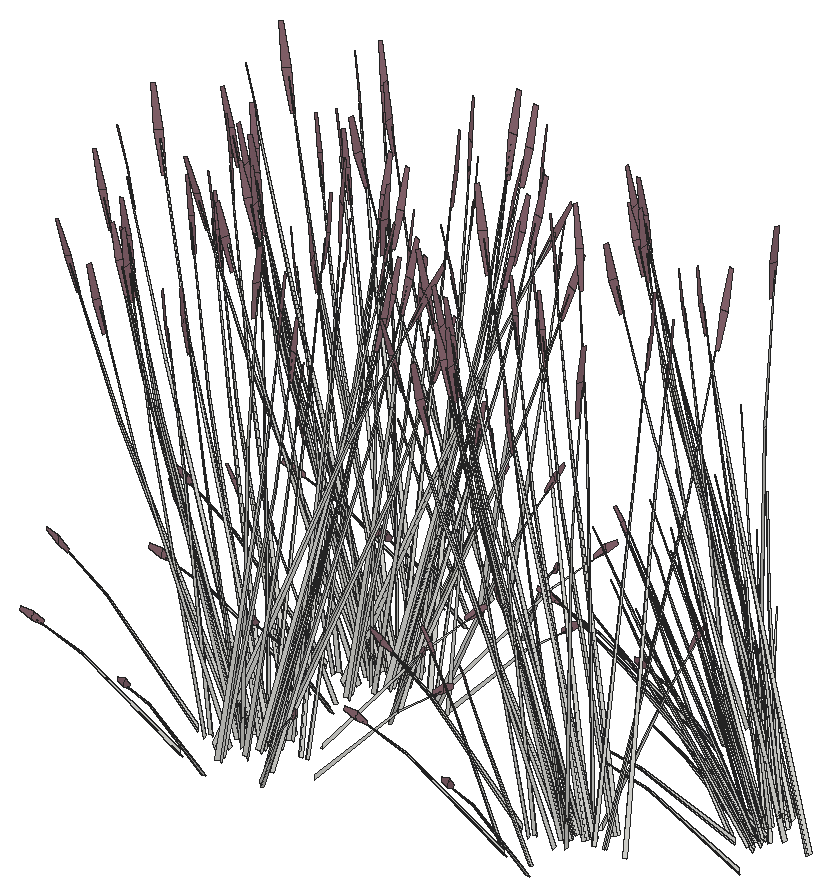
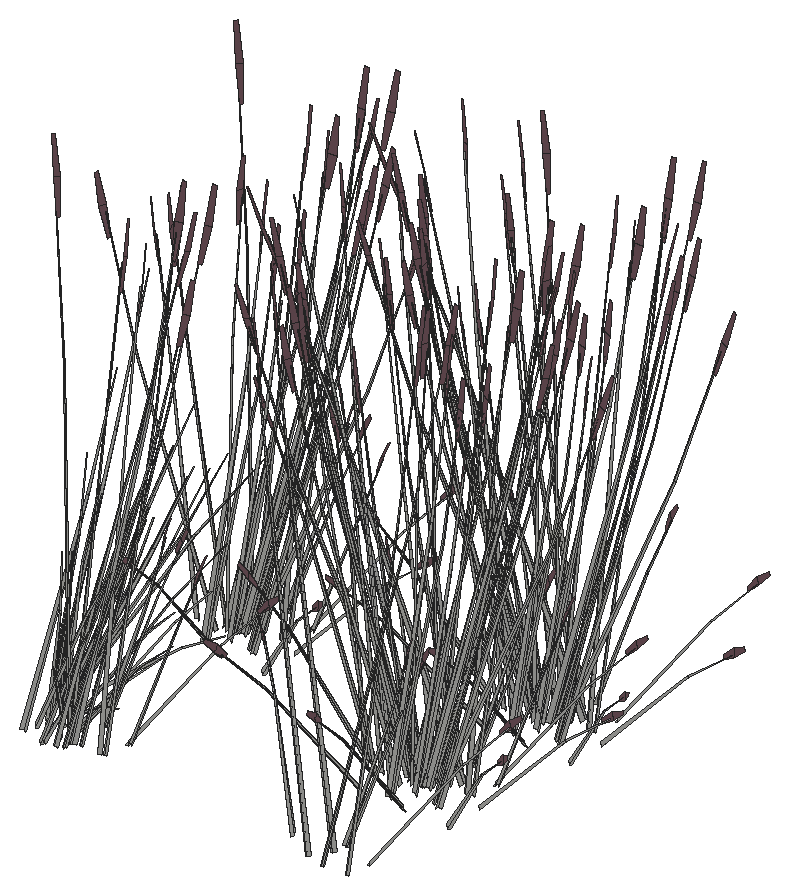
# SketchUp Ruby script. Lengths in inches.
U = 1.inch
M = Sketchup.active_model
def pt(a) = Geom::Point3d.new(a.map { |v| v * U })
def face(e, loops, mat)
  f = e.add_face(loops[0].map { |a| pt(a) })
  loops[1..].each { |l| e.add_face(l.map { |a| pt(a) }).erase! }
  f.material = f.back_material = mat if mat
  f
end
# faces: each face lists its corners as indices into pts; further lists are holes
def faces(e, pts, list, mat = nil) = list.each { |f| face(e, (f[0].is_a?(Array) ? f : [f]).map { |l| l.map { |i| pts[i] } }, mat) }
# xy, xz, yz: faces in a plane at the given z, y or x. An outline is a flat list of corners, or four numbers for a rectangle; further outlines are holes
def ring(l) = l.size == 4 ? [[l[0], l[1]], [l[2], l[1]], [l[2], l[3]], [l[0], l[3]]] : l.each_slice(2).to_a
def flat(e, list, mat, &to3) = list.each { |f| face(e, (f[0].is_a?(Array) ? f : [f]).map { |l| ring(l).map { |u, v| to3.(u, v) } }, mat) }
def xy(e, z, list, mat = nil) = flat(e, list, mat) { |x, y| [x, y, z] }
def xz(e, y, list, mat = nil) = flat(e, list, mat) { |x, z| [x, y, z] }
def yz(e, x, list, mat = nil) = flat(e, list, mat) { |y, z| [x, y, z] }
def lines(e, pts, list) = list.each { |a, b| e.add_line(pt(pts[a]), pt(pts[b])) }
# prism: a flat outline (further loops are holes) pulled along v
def prism(e, loops, v, mat = nil)
  f = face(e, loops, mat); d = Geom::Vector3d.new(v.map { |x| x * U })
  f.pushpull(f.normal.samedirection?(d) ? d.length : -d.length)
end
def box(e, o, s, mat = nil) = prism(e, [[o, [o[0] + s[0], o[1], o[2]], [o[0] + s[0], o[1] + s[1], o[2]], [o[0], o[1] + s[1], o[2]]]], [0, 0, s[2]], mat)
def at(x, y, z, deg = 0) = Geom::Transformation.translation(pt([x, y, z])) * Geom::Transformation.rotation(ORIGIN, Z_AXIS, deg.degrees)
def axes(o, x, y, z) = Geom::Transformation.new([*x, 0, *y, 0, *z, 0, *pt(o).to_a, 1])
def part(name) = M.definitions.add(name)
# library, detail: a bought-in or finely detailed component or shape, given as its bounding box
def library(name, o, s) = part(name).tap { |d| box(d.entities, o, s) }
def detail(e, o, s) = box(e.add_group.entities, o, s)
def put(e, d, t, mat = nil) = e.add_instance(d, t).tap { |i| i.material = mat if mat }
def group(e, t, mat = nil) = e.add_group.tap { |g| g.transformation = t; g.material = mat if mat }.entities
root = M.entities
M.materials.add("LightPink_Translucent").color = [144, 107, 117]
c1 = part("blade")
p = [[2.15,0.21,22],[0,0.17,0],[0.09,0.45,0],[2.18,0.31,22],[2.29,0.31,22],[0.38,0.45,0],
  [2.48,0.24,33],[2.49,0.24,33],[2.48,0.22,33]]
faces(c1.entities,p,[[0,1,2,3],[4,5,2,3],[6,3,4,7],[8,0,3,6]])
c2 = part("seeds")
p = [[0.3,-0.1,1.38],[-0.01,-0.03,1.59],[-0.01,-0.03,0.03],[0.14,-0.07,-0.07],[0.29,-0.03,3],[0.15,0.01,3.11]]
faces(c2.entities,p,[[0,1,2,3],[1,0,4,5]],"LightPink_Translucent")
c3 = part("blade with seeds")
put(c3.entities,c1,at(0,0,0))
put(c3.entities,c2,axes([2.4,0.25,30.99],[1.5799,-0.05474,1.17369],[-0.12525,1.92788,0.29478],[-0.07173,-0.02425,1.56792]))
c4 = part("blade with seeds\#1")
put(c4.entities,c1,at(0,0,0))
put(root,c3,axes([24.625,21.875,43.74],[0.03108,0.16322,1.76342],[-0.62654,0.85237,-0.26939],[-0.44504,-0.04296,0.30037]))
put(root,c3,axes([24.29,26.44,43.74],[0.16438,0.10347,1.76342],[0.27873,0.95868,-0.26939],[-0.36432,0.20444,0.30037]))
put(root,c3,axes([26.17,37.93,43.49],[0.03108,0.16322,1.76342],[-0.62654,0.85237,-0.26939],[-0.44504,-0.04296,0.30037]))
put(root,c3,axes([25.83,42.51,43.49],[0.16438,0.10347,1.76342],[0.27873,0.95868,-0.26939],[-0.36432,0.20444,0.30037]))
put(root,c3,axes([28.72,23.35,44.31],[-1.27479,-0.1698,-0.62353],[0.26901,-1.04736,-0.16365],[-0.38043,-0.12691,1.37633]))
put(root,c3,axes([27.05,25.34,44.27],[-1.14694,-0.51783,-0.49651],[0.68554,-0.92854,0],[-0.26122,-0.11794,1.57504]))
put(root,c3,axes([26.55,17.62,43.74],[-0.11871,0.13643,1.76342],[-1.19964,0.29415,-0.26939],[-0.2898,-0.26759,0.30037]))
put(root,c3,axes([30.27,39.41,44.06],[-1.27479,-0.1698,-0.62353],[0.26901,-1.04736,-0.16365],[-0.38043,-0.12691,1.37633]))
put(root,c3,axes([27.79,52.71,43.49],[-0.11871,0.13643,1.76342],[-1.19964,0.29415,-0.26939],[-0.2898,-0.26759,0.30037]))
put(root,c3,axes([28.59,41.4,44.02],[-1.14694,-0.51783,-0.49651],[0.68554,-0.92854,0],[-0.26122,-0.11794,1.57504]))
put(root,c3,axes([28.09,33.68,43.49],[-0.11871,0.13643,1.76342],[-1.19964,0.29415,-0.26939],[-0.2898,-0.26759,0.30037]))
put(root,c3,axes([30.17,23.51,44.92],[-1.23732,0.68758,-0.29095],[-0.8228,-0.97154,-0.50002],[-0.30528,-0.09867,1.59708]))
put(root,c3,axes([27.37,24.95,44.28],[-0.28787,-0.90242,-0.30978],[1.14332,-0.25625,0.30978],[-0.23049,-0.10406,1.38974]))
put(root,c3,axes([30.99,24.26,44.31],[-0.82544,0.77843,-0.62353],[-1.0254,-0.70586,-0.16365],[-0.33076,0.19418,1.37633]))
put(root,c3,axes([27.34,34.21,44.13],[-0.35352,0.84566,-0.03893],[-1.08806,-0.26014,-0.17649],[-0.1652,-0.13832,0.58215]))
put(root,c3,axes([31.56,23.82,44.72],[-1.19666,-0.83357,-0.25192],[1.00694,-0.93603,0.5513],[-0.32224,0.09751,1.68216]))
put(root,c3,axes([31.71,39.57,44.67],[-1.23732,0.68758,-0.29095],[-0.8228,-0.97154,-0.50002],[-0.30528,-0.09867,1.59708]))
put(root,c3,axes([29.38,23.02,44.46],[-0.73619,-0.86927,-0.44739],[1.11511,-0.61213,0.21531],[-0.23824,-0.10756,1.43643]))
put(root,c3,axes([28.91,41.01,44.03],[-0.28787,-0.90242,-0.30978],[1.14332,-0.25625,0.30978],[-0.23049,-0.10406,1.38974]))
put(root,c3,axes([30.95,23.64,44.46],[-1.33077,0.06393,-0.44739],[-0.12035,-1.06125,0.21531],[-0.23824,0.10756,1.43643]))
put(root,c3,axes([32.53,40.32,44.06],[-0.82544,0.77843,-0.62353],[-1.0254,-0.70586,-0.16365],[-0.33076,0.19418,1.37633]))
put(root,c3,axes([33.1,39.88,44.46],[-1.19666,-0.83357,-0.25192],[1.00694,-0.93603,0.5513],[-0.32224,0.09751,1.68216]))
put(root,c3,axes([30.93,39.08,44.21],[-0.73619,-0.86927,-0.44739],[1.11511,-0.61213,0.21531],[-0.23824,-0.10756,1.43643]))
put(root,c3,axes([32.35,26.38,44.27],[-1.14694,0.51783,-0.49651],[-0.68554,-0.92854,0],[-0.26122,0.11794,1.57504]))
put(root,c3,axes([25.56,21.22,44.27],[0,-1.03566,-0.49651],[1.37109,0,0],[0,-0.23588,1.57504]))
put(root,c3,axes([32.5,39.7,44.21],[-1.33077,0.06393,-0.44739],[-0.12035,-1.06125,0.21531],[-0.23824,0.10756,1.43643]))
put(root,c3,axes([32.08,25.97,44.28],[-1.14332,-0.25625,-0.30978],[0.28787,-0.90242,0.30978],[-0.23049,0.10406,1.38974]))
put(root,c3,axes([29.14,22.42,44.92],[-1.38012,-0.49416,-0.29095],[0.66454,-1.04299,-0.50002],[-0.04337,-0.25608,1.59708]))
put(root,c3,axes([31.03,39.58,44.4375],[0.32481,-1.2272,-0.23429],[1.54007,0.21392,0.51271],[-0.26911,-0.16947,1.5644]))
put(root,c3,axes([31.88,23.36,44.92],[0.1428,1.18174,-0.29095],[-1.48733,0.07145,-0.50002],[-0.26191,0.15741,1.59708]))
put(root,c3,axes([26.8,56.3125,44.02],[0,-1.03566,-0.49651],[1.37109,0,0],[0,-0.23588,1.57504]))
put(root,c3,axes([28.53,21.37,44.35],[-0.50328,-1.06202,-0.69835],[1.44974,-0.38248,-0.18329],[-0.05563,-0.35963,1.54149]))
put(root,c3,axes([33.89,42.44,44.02],[-1.14694,0.51783,-0.49651],[-0.68554,-0.92854,0],[-0.26122,0.11794,1.57504]))
put(root,c3,axes([27.1,37.28,44.02],[0,-1.03566,-0.49651],[1.37109,0,0],[0,-0.23588,1.57504]))
put(root,c3,axes([26.15,21.25,44.28],[0.85545,-0.64616,-0.30978],[0.85545,0.64616,0.30978],[0,-0.20813,1.38974]))
put(root,c3,axes([33.625,42.03,44.03],[-1.14332,-0.25625,-0.30978],[0.28787,-0.90242,0.30978],[-0.23049,0.10406,1.38974]))
put(root,c3,axes([30.6875,38.48,44.67],[-1.38012,-0.49416,-0.29095],[0.66454,-1.04299,-0.50002],[-0.04337,-0.25608,1.59708]))
put(root,c3,axes([29.77,56.46,44.1],[-0.50328,-1.06202,-0.69835],[1.44974,-0.38248,-0.18329],[-0.05563,-0.35963,1.54149]))
put(root,c3,axes([33.43,39.42,44.67],[0.1428,1.18174,-0.29095],[-1.48733,0.07145,-0.50002],[-0.26191,0.15741,1.59708]))
put(root,c3,axes([30.07,37.43,44.1],[-0.50328,-1.06202,-0.69835],[1.44974,-0.38248,-0.18329],[-0.05563,-0.35963,1.54149]))
put(root,c3,axes([31.26,52.16,44.13],[-0.84686,0.59414,-0.03893],[-0.77596,-0.65071,-0.17649],[-0.05463,-0.18438,0.58215]))
put(root,c3,axes([27.69,37.31,44.03],[0.85545,-0.64616,-0.30978],[0.85545,0.64616,0.30978],[0,-0.20813,1.38974]))
put(root,c3,axes([31.55,33.13,44.13],[-0.84686,0.59414,-0.03893],[-0.77596,-0.65071,-0.17649],[-0.05463,-0.18438,0.58215]))
put(root,c3,axes([30.22,16.34,43.74],[-0.20555,0.03731,1.76342],[-1.13672,-0.42002,-0.26939],[0.01907,-0.35034,0.30037]))
put(root,c3,axes([29.29,21.65,44.46],[0.59459,-0.93321,-0.44739],[1.23546,0.44912,0.21531],[0,-0.21512,1.43643]))
put(root,c3,axes([29.36,26.54,43.74],[0.19833,-0.05635,1.76342],[1.19302,0.31018,-0.26939],[0.03489,0.3496,0.30037]))
put(root,c3,axes([31.47,51.43,43.49],[-0.20555,0.03731,1.76342],[-1.13672,-0.42002,-0.26939],[0.01907,-0.35034,0.30037]))
put(root,c3,axes([32.43,22.89,44.46],[-0.59459,0.93321,-0.44739],[-1.23546,-0.44912,0.21531],[0,0.21512,1.43643]))
put(root,c3,axes([31.77,32.4,43.49],[-0.20555,0.03731,1.76342],[-1.13672,-0.42002,-0.26939],[0.01907,-0.35034,0.30037]))
put(root,c3,axes([30.83,37.71,44.21],[0.59459,-0.93321,-0.44739],[1.23546,0.44912,0.21531],[0,-0.21512,1.43643]))
put(root,c3,axes([30.91,42.6,43.49],[0.19833,-0.05635,1.76342],[1.19302,0.31018,-0.26939],[0.03489,0.3496,0.30037]))
put(root,c3,axes([33.97,38.95,44.21],[-0.59459,0.93321,-0.44739],[-1.23546,-0.44912,0.21531],[0,0.21512,1.43643]))
put(root,c3,axes([35.57,23.29,44.28],[-0.85545,0.64616,-0.30978],[-0.85545,-0.64616,0.30978],[0,0.20813,1.38974]))
put(root,c3,axes([33.125,23.18,44.35],[0.44936,0.94823,-0.69212],[-1.29441,0.3415,-0.18165],[0.04967,0.32109,1.52773]))
put(root,c3,axes([29.83,21.18,44.92],[-0.1428,-1.18174,-0.29095],[1.48733,-0.07145,-0.50002],[0.26191,-0.15741,1.59708]))
put(root,c3,axes([32.57,22.12,44.92],[1.38012,0.49416,-0.29095],[-0.66454,1.04299,-0.50002],[0.04337,0.25608,1.59708]))
put(root,c3,axes([29.64,18.57,44.28],[1.14332,0.25625,-0.30978],[-0.28787,0.90242,0.30978],[0.23049,-0.10406,1.38974]))
put(root,c3,axes([37.12,39.35,44.03],[-0.85545,0.64616,-0.30978],[-0.85545,-0.64616,0.30978],[0,0.20813,1.38974]))
put(root,c3,axes([36.16,23.32,44.27],[0,1.03566,-0.49651],[-1.37109,0,0],[0,0.23588,1.57504]))
put(root,c3,axes([29.37,18.16,44.27],[1.14694,-0.51783,-0.49651],[0.68554,0.92854,0],[0.26122,-0.11794,1.57504]))
put(root,c3,axes([34.67,39.24,44.09],[0.44936,0.94823,-0.69212],[-1.29441,0.3415,-0.18165],[0.04967,0.32109,1.52773]))
put(root,c3,axes([31.38,37.24,44.67],[-0.1428,-1.18174,-0.29095],[1.48733,-0.07145,-0.50002],[0.26191,-0.15741,1.59708]))
put(root,c3,axes([34.12,38.18,44.67],[1.38012,0.49416,-0.29095],[-0.66454,1.04299,-0.50002],[0.04337,0.25608,1.59708]))
put(root,c3,axes([32.31,24.53,44.4375],[1.2866,-0.3514,-0.19198],[0.45209,1.01223,0.00008],[0.14202,-0.03884,1.73897]))
put(root,c3,axes([31.18,34.63,44.03],[1.14332,0.25625,-0.30978],[-0.28787,0.90242,0.30978],[0.23049,-0.10406,1.38974]))
put(root,c3,axes([30.61,53.25,44.02],[1.14694,-0.51783,-0.49651],[0.68554,0.92854,0],[0.26122,-0.11794,1.57504]))
put(root,c3,axes([37.7,39.38,44.02],[0,1.03566,-0.49651],[-1.37109,0,0],[0,0.23588,1.57504]))
put(root,c3,axes([30.91,34.22,44.02],[1.14694,-0.51783,-0.49651],[0.68554,0.92854,0],[0.26122,-0.11794,1.57504]))
put(root,c3,axes([32.33,21.52,44.46],[0.73619,0.86927,-0.44739],[-1.11511,0.61213,0.21531],[0.23824,0.10756,1.43643]))
put(root,c3,axes([30.73,20.28,44.31],[0.82544,-0.77843,-0.62353],[1.0254,0.70586,-0.16365],[0.33076,-0.19418,1.37633]))
put(root,c3,axes([33.85,40.59,44.18],[1.2866,-0.3514,-0.19198],[0.45209,1.01223,0.00008],[0.14202,-0.03884,1.73897]))
put(root,c3,axes([34.35,19.59,44.28],[0.28787,0.90242,-0.30978],[-1.14332,0.25625,0.30978],[0.23049,0.10406,1.38974]))
put(root,c3,axes([33.88,37.58,44.21],[0.73619,0.86927,-0.44739],[-1.11511,0.61213,0.21531],[0.23824,0.10756,1.43643]))
put(root,c3,axes([31.55,21.03,44.92],[1.23732,-0.68758,-0.29095],[0.8228,0.97154,-0.50002],[0.30528,0.09867,1.59708]))
put(root,c3,axes([31.97,55.37,44.06],[0.82544,-0.77843,-0.62353],[1.0254,0.70586,-0.16365],[0.33076,-0.19418,1.37633]))
put(root,c3,axes([32.27,36.34,44.06],[0.82544,-0.77843,-0.62353],[1.0254,0.70586,-0.16365],[0.33076,-0.19418,1.37633]))
put(root,c3,axes([28.43,20.42,43.84],[-1.20625,0.41464,1.28929],[-0.38394,-1.1897,0.50096],[0.74071,0.01979,1.46642]))
put(root,c3,axes([35.89,35.65,44.03],[0.28787,0.90242,-0.30978],[-1.14332,0.25625,0.30978],[0.23049,0.10406,1.38974]))
put(root,c3,axes([33.09,37.09,44.67],[1.23732,-0.68758,-0.29095],[0.8228,0.97154,-0.50002],[0.30528,0.09867,1.59708]))
put(root,c3,axes([35.25,18.125,43.74],[-0.18342,-0.08159,1.76342],[-0.47115,-0.9115,-0.26939],[0.31784,-0.24736,0.30037]))
put(root,c3,axes([34.67,19.2,44.27],[1.14694,0.51783,-0.49651],[-0.68554,0.92854,0],[0.26122,0.11794,1.57504]))
put(root,c3,axes([34.61,26.57,43.74],[0.08928,-0.14952,1.76342],[1.12407,-0.44035,-0.26939],[0.34078,0.22791,0.30037]))
put(root,c3,axes([29.97,36.48,43.59],[-1.20625,0.41464,1.28929],[-0.38394,-1.1897,0.50096],[0.74071,0.01979,1.46642]))
put(root,c3,axes([33,21.1875,44.31],[1.27479,0.1698,-0.62353],[-0.26901,1.04736,-0.16365],[0.38043,0.12691,1.37633]))
put(root,c3,axes([36.5,53.22,43.49],[-0.18342,-0.08159,1.76342],[-0.47115,-0.9115,-0.26939],[0.31784,-0.24736,0.30037]))
put(root,c3,axes([36.8,34.1875,43.49],[-0.18342,-0.08159,1.76342],[-0.47115,-0.9115,-0.26939],[0.31784,-0.24736,0.30037]))
put(root,c3,axes([36.21,35.26,44.02],[1.14694,0.51783,-0.49651],[-0.68554,0.92854,0],[0.26122,0.11794,1.57504]))
put(root,c3,axes([36.16,42.63,43.49],[0.08928,-0.14952,1.76342],[1.12407,-0.44035,-0.26939],[0.34078,0.22791,0.30037]))
put(root,c3,axes([34.54,37.25,44.06],[1.27479,0.1698,-0.62353],[-0.26901,1.04736,-0.16365],[0.38043,0.12691,1.37633]))
put(root,c3,axes([39.97,37.86,44.26],[-0.75977,-0.66224,-0.06488],[0.83212,-0.6068,-0.29416],[0.23578,-0.04272,0.97024]))
put(root,c3,axes([37.85,22.03,43.74],[-0.06405,-0.15723,1.76342],[0.44421,-0.91974,-0.26939],[0.4481,-0.01323,0.30037]))
put(root,c3,axes([38.53,38.74,43.98],[-0.7893,0.12429,1.41583],[-0.12563,-0.9893,0.08104],[0.55282,-0.14974,0.80566]))
put(root,c3,axes([39.39,38.09,43.49],[-0.06405,-0.15723,1.76342],[0.44421,-0.91974,-0.26939],[0.4481,-0.01323,0.30037]))
put(root,c3,axes([57.64,25.93,43.49],[0.03108,0.16322,1.76342],[-0.62654,0.85237,-0.26939],[-0.44504,-0.04296,0.30037]))
put(root,c3,axes([57.3,30.51,43.49],[0.16438,0.10347,1.76342],[0.27873,0.95868,-0.26939],[-0.36432,0.20444,0.30037]))
put(root,c3,axes([61.74,27.41,44.06],[-1.27479,-0.1698,-0.62353],[0.26901,-1.04736,-0.16365],[-0.38043,-0.12691,1.37633]))
put(root,c3,axes([59.35,48.97,43.49],[-0.11871,0.13643,1.76342],[-1.19964,0.29415,-0.26939],[-0.2898,-0.26759,0.30037]))
put(root,c3,axes([60.07,29.4,44.02],[-1.14694,-0.51783,-0.49651],[0.68554,-0.92854,0],[-0.26122,-0.11794,1.57504]))
put(root,c3,axes([59.5625,21.68,43.49],[-0.11871,0.13643,1.76342],[-1.19964,0.29415,-0.26939],[-0.2898,-0.26759,0.30037]))
put(root,c3,axes([58.61,49.49,44.13],[-0.35352,0.84566,-0.03893],[-1.08806,-0.26014,-0.17649],[-0.1652,-0.13832,0.58215]))
put(root,c3,axes([58.82,22.21,44.13],[-0.35352,0.84566,-0.03893],[-1.08806,-0.26014,-0.17649],[-0.1652,-0.13832,0.58215]))
put(root,c3,axes([63.18,27.57,44.67],[-1.23732,0.68758,-0.29095],[-0.8228,-0.97154,-0.50002],[-0.30528,-0.09867,1.59708]))
put(root,c3,axes([60.39,29.01,44.03],[-0.28787,-0.90242,-0.30978],[1.14332,-0.25625,0.30978],[-0.23049,-0.10406,1.38974]))
put(root,c3,axes([64.01,28.32,44.06],[-0.82544,0.77843,-0.62353],[-1.0254,-0.70586,-0.16365],[-0.33076,0.19418,1.37633]))
put(root,c3,axes([62.19,54.37,44.21],[-0.73619,-0.86927,-0.44739],[1.11511,-0.61213,0.21531],[-0.23824,-0.10756,1.43643]))
put(root,c3,axes([64.57,27.88,44.46],[-1.19666,-0.83357,-0.25192],[1.00694,-0.93603,0.5513],[-0.32224,0.09751,1.68216]))
put(root,c3,axes([62.4,27.08,44.21],[-0.73619,-0.86927,-0.44739],[1.11511,-0.61213,0.21531],[-0.23824,-0.10756,1.43643]))
put(root,c3,axes([63.97,27.7,44.21],[-1.33077,0.06393,-0.44739],[-0.12035,-1.06125,0.21531],[-0.23824,0.10756,1.43643]))
put(root,c3,axes([62.3,54.87,44.4375],[0.32481,-1.2272,-0.23429],[1.54007,0.21392,0.51271],[-0.26911,-0.16947,1.5644]))
put(root,c3,axes([62.51,27.58,44.4375],[0.32481,-1.2272,-0.23429],[1.54007,0.21392,0.51271],[-0.26911,-0.16947,1.5644]))
put(root,c3,axes([58.37,52.57,44.02],[0,-1.03566,-0.49651],[1.37109,0,0],[0,-0.23588,1.57504]))
put(root,c3,axes([65.37,30.44,44.02],[-1.14694,0.51783,-0.49651],[-0.68554,-0.92854,0],[-0.26122,0.11794,1.57504]))
put(root,c3,axes([58.58,25.28,44.02],[0,-1.03566,-0.49651],[1.37109,0,0],[0,-0.23588,1.57504]))
put(root,c3,axes([61.95,53.77,44.67],[-1.38012,-0.49416,-0.29095],[0.66454,-1.04299,-0.50002],[-0.04337,-0.25608,1.59708]))
put(root,c3,axes([65.1,30.03,44.03],[-1.14332,-0.25625,-0.30978],[0.28787,-0.90242,0.30978],[-0.23049,0.10406,1.38974]))
put(root,c3,axes([62.16,26.48,44.67],[-1.38012,-0.49416,-0.29095],[0.66454,-1.04299,-0.50002],[-0.04337,-0.25608,1.59708]))
put(root,c3,axes([61.33,52.72,44.1],[-0.50328,-1.06202,-0.69835],[1.44974,-0.38248,-0.18329],[-0.05563,-0.35963,1.54149]))
put(root,c3,axes([64.9,27.42,44.67],[0.1428,1.18174,-0.29095],[-1.48733,0.07145,-0.50002],[-0.26191,0.15741,1.59708]))
put(root,c3,axes([61.54,25.43,44.1],[-0.50328,-1.06202,-0.69835],[1.44974,-0.38248,-0.18329],[-0.05563,-0.35963,1.54149]))
put(root,c3,axes([58.95,52.59,44.03],[0.85545,-0.64616,-0.30978],[0.85545,0.64616,0.30978],[0,-0.20813,1.38974]))
put(root,c3,axes([62.82,48.41,44.13],[-0.84686,0.59414,-0.03893],[-0.77596,-0.65071,-0.17649],[-0.05463,-0.18438,0.58215]))
put(root,c3,axes([59.16,25.31,44.03],[0.85545,-0.64616,-0.30978],[0.85545,0.64616,0.30978],[0,-0.20813,1.38974]))
put(root,c3,axes([63.03,21.13,44.13],[-0.84686,0.59414,-0.03893],[-0.77596,-0.65071,-0.17649],[-0.05463,-0.18438,0.58215]))
put(root,c3,axes([63.03,47.6875,43.49],[-0.20555,0.03731,1.76342],[-1.13672,-0.42002,-0.26939],[0.01907,-0.35034,0.30037]))
put(root,c3,axes([63.24,20.4,43.49],[-0.20555,0.03731,1.76342],[-1.13672,-0.42002,-0.26939],[0.01907,-0.35034,0.30037]))
put(root,c3,axes([62.1,52.99,44.21],[0.59459,-0.93321,-0.44739],[1.23546,0.44912,0.21531],[0,-0.21512,1.43643]))
put(root,c3,axes([62.31,25.71,44.21],[0.59459,-0.93321,-0.44739],[1.23546,0.44912,0.21531],[0,-0.21512,1.43643]))
put(root,c4,axes([71.11,46.72,40.07],[0.31369,-0.26428,1.54493],[0.26409,1.22118,0.12492],[-0.49247,0.276,0.66044]))
put(root,c4,axes([69.03,44.71,40.82],[-0.13699,0.17683,1.57709],[0.08685,1.18009,-0.24942],[-0.32765,0.18834,0.12648]))
put(root,c3,axes([62.38,30.6,43.49],[0.19833,-0.05635,1.76342],[1.19302,0.31018,-0.26939],[0.03489,0.3496,0.30037]))
put(root,c4,axes([70.65,41.97,38.91],[0.19776,0.32863,1.28914],[-0.34614,0.98419,-0.27724],[-0.43048,-0.18244,0.55117]))
put(root,c4,axes([71.34,43.47,41.0625],[-0.79444,0.5518,-0.64046],[-0.44274,-1.13586,0.07729],[-0.38385,0.12903,0.906]))
put(root,c4,axes([70.28,47.06,38.91],[0.31962,0.07001,1.28914],[0.26756,1.02347,-0.27724],[-0.41311,0.23924,0.55117]))
put(root,c4,axes([69.58,44.42,37.92],[0.0352,0.19392,1.5897],[-0.39624,1.07238,-0.24285],[-0.33051,-0.01799,0.27078]))
put(root,c3,axes([65.44,26.95,44.21],[-0.59459,0.93321,-0.44739],[-1.23546,-0.44912,0.21531],[0,0.21512,1.43643]))
put(root,c4,axes([70.01,39.66,40.82],[0.07463,0.11741,1.59908],[-0.25178,1.15035,-0.1511],[-0.32567,0.04164,0.28298]))
put(root,c4,axes([70.71,39.41,40.82],[-0.19445,0.01116,1.57709],[-0.562,0.94258,-0.24942],[-0.34067,-0.14573,0.12648]))
put(root,c4,axes([72.12,41.17,41.0625],[-0.90375,-0.03008,-0.64046],[0.0607,-1.26677,0.07729],[-0.38287,-0.13368,0.906]))
put(root,c4,axes([71.66,42.6,40.07],[0.33582,0.21526,1.54493],[-0.69497,0.90306,0.12492],[-0.43315,-0.40739,0.66044]))
put(root,c4,axes([70.67,43.37,40.65],[-0.75135,-0.34854,-0.31925],[0.21915,-1.01686,0.41216],[-0.30251,0.09324,0.78863]))
put(root,c4,axes([69.08,43.18,39.07],[0.56973,-0.14831,1.03545],[-0.31555,0.82274,0.76078],[-0.29172,-0.08853,0.22807]))
put(root,c4,axes([71.18,43.88,40.79],[-0.24493,1.13649,-0.46065],[-0.83975,-0.38955,-0.35681],[-0.33809,0.10421,0.88141]))
put(root,c4,axes([68.58,45.92,40.82],[0.11711,0.02157,1.59908],[0.42502,1.06376,-0.1511],[-0.21726,0.31303,0.28298]))
put(root,c4,axes([71.82,41.43,40.79],[-0.65648,0.82762,-0.46065],[-0.57493,-0.87428,-0.35681],[-0.33354,-0.12593,0.88141]))
put(root,c4,axes([71.14,42.91,41.11],[0.45489,1.13134,-0.10962],[-0.80735,0.55596,-0.60845],[-0.34022,0.14927,0.92453]))
put(root,c4,axes([70.66,46.15,41.17],[-0.25113,-1.28788,0.48466],[0.9851,-0.22351,0.39963],[-0.29033,0.30289,1.00289]))
put(root,c4,axes([69.76,47.41,39.07],[0.34005,-0.60308,1.03545],[0.20441,0.87829,0.76078],[-0.26134,0.18792,0.22807]))
put(root,c4,axes([70.84,43.24,40.84],[0.25543,-1.1392,0.43274],[0.83975,0.38955,0.35681],[-0.33023,0.06846,0.89544]))
put(root,c4,axes([72.16,40.5625,41.11],[-0.04841,1.27062,-0.10962],[-0.91657,-0.03473,-0.60845],[-0.353,-0.08826,0.92453]))
put(root,c4,axes([70.78,42.9375,40.84],[-0.33205,-0.8519,0.05797],[0.60551,-0.41697,0.45634],[-0.26692,0.08227,0.69585]))
put(root,c4,axes([70.94,46.3,40.65],[-0.78697,0.17856,-0.31925],[-0.2078,-1.02074,0.41216],[-0.22552,0.27417,0.78863]))
put(root,c4,axes([71.58,40.65,40.65],[-0.51441,-0.78225,-0.31925],[0.58738,-0.7405,0.41216],[-0.29843,-0.11267,0.78863]))
put(root,c4,axes([70.87,45.86,40.84],[-0.62066,-0.52545,0.05797],[0.36135,-0.74826,0.45634],[-0.19899,0.24191,0.69585]))
put(root,c4,axes([71.26,39.67,37.92],[-0.07697,0.17304,1.5897],[-0.85991,0.44448,-0.24285],[-0.23336,-0.29985,0.27078]))
put(root,c3,axes([68.59,27.35,44.03],[-0.85545,0.64616,-0.30978],[-0.85545,-0.64616,0.30978],[0,0.20813,1.38974]))
put(root,c4,axes([71.46,43.25,41.13],[0.75135,0.34854,0.31925],[-0.21915,1.01686,-0.41216],[-0.30251,0.09324,0.78863]))
put(root,c4,axes([74.33,46.02,38.47],[-1.0019,0.47479,-0.62955],[-0.36083,-1.36768,-0.16523],[-0.33927,0.05248,1.38963]))
put(root,c3,axes([66.14,27.24,44.09],[0.44936,0.94823,-0.69212],[-1.29441,0.3415,-0.18165],[0.04967,0.32109,1.52773]))
put(root,c3,axes([62.64,52.53,44.67],[-0.1428,-1.18174,-0.29095],[1.48733,-0.07145,-0.50002],[0.26191,-0.15741,1.59708]))
put(root,c4,axes([71.78,40.65,40.84],[0.66663,-0.82326,0.43274],[0.57493,0.87428,0.35681],[-0.31276,-0.15186,0.89544]))
put(root,c3,axes([62.85,25.24,44.67],[-0.1428,-1.18174,-0.29095],[1.48733,-0.07145,-0.50002],[0.26191,-0.15741,1.59708]))
put(root,c4,axes([71.84,40.35,40.84],[0.04552,-0.95007,0.05797],[0.68742,0.02605,0.45634],[-0.26332,-0.09941,0.69585]))
put(root,c4,axes([72.3,41.06,41.13],[0.51441,0.78225,0.31925],[-0.58738,0.7405,-0.41216],[-0.29843,-0.11267,0.78863]))
put(root,c4,axes([70.27,44.62,38.49],[0.56051,0.79893,-0.03509],[-0.61388,0.73204,-0.15911],[-0.17394,0.05154,0.52479]))
put(root,c4,axes([71.45,46.21,38.71],[-0.97904,0.72283,0],[-0.54599,-1.20931,-0.46523],[-0.12435,-0.27543,1.47583]))
